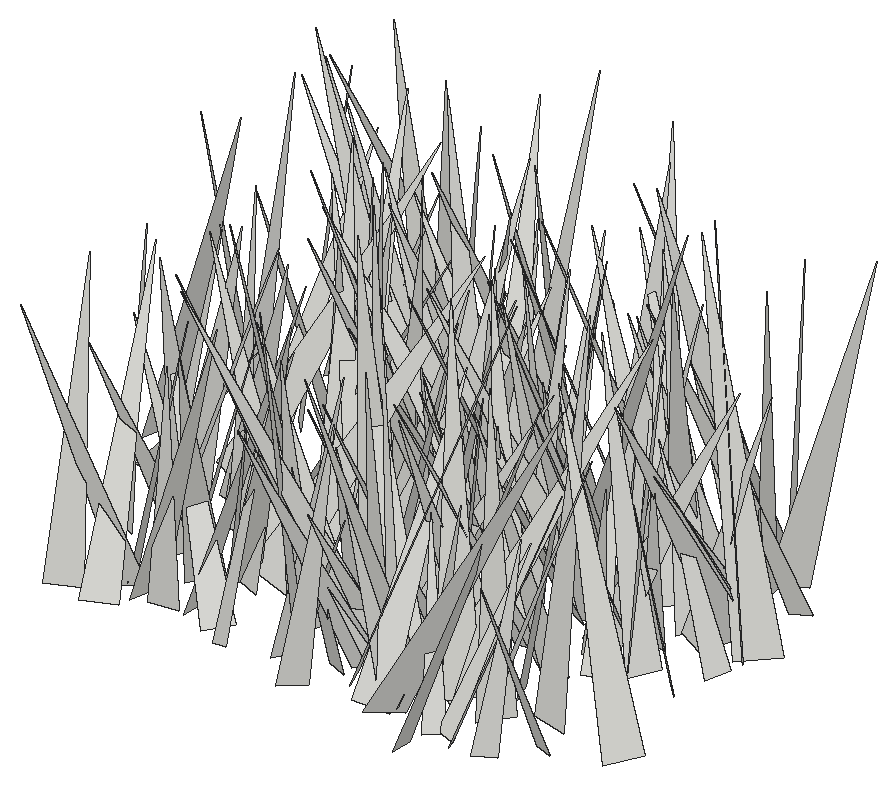
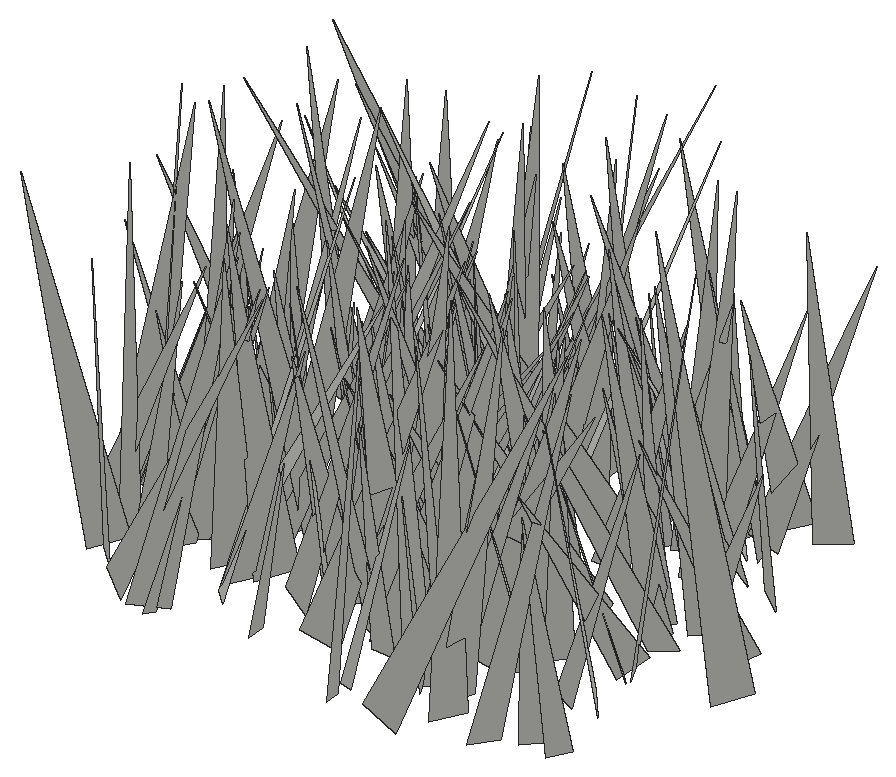
# SketchUp Ruby script. Lengths in inches.
U = 1.inch
M = Sketchup.active_model
def pt(a) = Geom::Point3d.new(a.map { |v| v * U })
def face(e, loops, mat)
  f = e.add_face(loops[0].map { |a| pt(a) })
  loops[1..].each { |l| e.add_face(l.map { |a| pt(a) }).erase! }
  f.material = f.back_material = mat if mat
  f
end
# faces: each face lists its corners as indices into pts; further lists are holes
def faces(e, pts, list, mat = nil) = list.each { |f| face(e, (f[0].is_a?(Array) ? f : [f]).map { |l| l.map { |i| pts[i] } }, mat) }
# xy, xz, yz: faces in a plane at the given z, y or x. An outline is a flat list of corners, or four numbers for a rectangle; further outlines are holes
def ring(l) = l.size == 4 ? [[l[0], l[1]], [l[2], l[1]], [l[2], l[3]], [l[0], l[3]]] : l.each_slice(2).to_a
def flat(e, list, mat, &to3) = list.each { |f| face(e, (f[0].is_a?(Array) ? f : [f]).map { |l| ring(l).map { |u, v| to3.(u, v) } }, mat) }
def xy(e, z, list, mat = nil) = flat(e, list, mat) { |x, y| [x, y, z] }
def xz(e, y, list, mat = nil) = flat(e, list, mat) { |x, z| [x, y, z] }
def yz(e, x, list, mat = nil) = flat(e, list, mat) { |y, z| [x, y, z] }
def lines(e, pts, list) = list.each { |a, b| e.add_line(pt(pts[a]), pt(pts[b])) }
# prism: a flat outline (further loops are holes) pulled along v
def prism(e, loops, v, mat = nil)
  f = face(e, loops, mat); d = Geom::Vector3d.new(v.map { |x| x * U })
  f.pushpull(f.normal.samedirection?(d) ? d.length : -d.length)
end
def box(e, o, s, mat = nil) = prism(e, [[o, [o[0] + s[0], o[1], o[2]], [o[0] + s[0], o[1] + s[1], o[2]], [o[0], o[1] + s[1], o[2]]]], [0, 0, s[2]], mat)
def at(x, y, z, deg = 0) = Geom::Transformation.translation(pt([x, y, z])) * Geom::Transformation.rotation(ORIGIN, Z_AXIS, deg.degrees)
def axes(o, x, y, z) = Geom::Transformation.new([*x, 0, *y, 0, *z, 0, *pt(o).to_a, 1])
def part(name) = M.definitions.add(name)
# library, detail: a bought-in or finely detailed component or shape, given as its bounding box
def library(name, o, s) = part(name).tap { |d| box(d.entities, o, s) }
def detail(e, o, s) = box(e.add_group.entities, o, s)
def put(e, d, t, mat = nil) = e.add_instance(d, t).tap { |i| i.material = mat if mat }
def group(e, t, mat = nil) = e.add_group.tap { |g| g.transformation = t; g.material = mat if mat }.entities
root = M.entities
c1 = part("fur_instance\#9")
p = [[0.8125,0,1.79],[0.67,-0.02,1.48],[0,-0.11,0],[0,0.11,0]]
faces(c1.entities,p,[[0,1,2,3]])
put(root,c1,axes([124.41,342.08,-27.1],[4.29417,-2.87763,1.75823],[-3.19183,-4.38696,0.6155],[-1.08829,1.5119,5.13243]))
put(root,c1,axes([124.15,342.98,-27.1],[-6.04607,-3.24149,2.31572],[-3.3744,6.40425,0.15438],[2.11738,0.95032,6.85845]))
put(root,c1,axes([125.6,344.76,-27.1],[1.43774,-5.64122,0.58152],[-5.34924,-1.54822,-1.79367],[-1.88339,0.09091,5.53834]))
put(root,c1,axes([133.97,343.88,-27.1],[-1.2303,-3.6424,0.32202],[-3.65502,1.23499,0.00478],[0.10759,0.30356,3.84457]))
put(root,c1,axes([132.68,342.28,-27.1],[-2.57998,2.99071,1.64125],[3.02202,2.95835,-0.64026],[1.58287,-0.77341,3.89753]))
put(root,c1,axes([126.14,345.06,-27.1],[-8.04638,-2.10125,0.20494],[-2.02323,7.90531,1.61682],[0.60315,-1.51404,8.15753]))
put(root,c1,axes([127.17,345.21,-27.1],[-6.19203,-3.31038,1.54754],[-2.85802,6.28451,2.00782],[2.2771,-1.114,6.72819]))
put(root,c1,axes([115.82,344.11,-27.1],[-0.4063,-5.76079,1.26429],[-5.69006,0.04941,-1.60344],[-1.5519,1.32705,5.54804]))
put(root,c1,axes([116.51,344.07,-27.1],[6.83641,-1.96558,0.32372],[-1.94381,-6.83529,-0.45298],[-0.43579,-0.34652,7.09893]))
put(root,c1,axes([117.53,343.63,-27.1],[1.49528,-4.80686,1.53266],[-5.04418,-1.45777,0.34917],[-0.10564,1.56838,5.02194]))
put(root,c1,axes([130.01,341.07,-27.1],[6.47636,2.00005,0.90058],[1.74291,-6.39683,1.67254],[-1.33173,1.35459,6.56857]))
put(root,c1,axes([127.65,343.46,-27.1],[-4.79801,0.15244,1.14259],[0.25589,4.91001,0.4195],[1.12396,-0.46714,4.78206]))
put(root,c1,axes([128.04,342.59,-27.1],[7.15691,-3.14413,0.26361],[-3.09126,-6.8566,2.14652],[0.63178,2.06831,7.5166]))
put(root,c1,axes([113.94,342.64,-27.1],[3.27303,-4.65782,3.06275],[-5.40234,-3.52629,0.41046],[-1.37496,2.76738,5.67799]))
put(root,c1,axes([130.34,342.45,-27.1],[-3.13044,2.30171,0.23571],[2.28042,3.13636,-0.34054],[0.39127,0.13578,3.8706]))
put(root,c1,axes([123.11,344.1,-27.1],[3.6641,-0.22277,0.06955],[-0.2117,-3.63329,-0.48425],[-0.09821,-0.47926,3.63879]))
put(root,c1,axes([117.4375,346.02,-27.1],[4.70982,-4.44224,0.12242],[-4.38661,-4.67586,-0.90827],[-0.71149,-0.57769,6.41023]))
put(root,c1,axes([125.21,346.05,-27.1],[3.98276,-1.20965,1.22676],[-0.42908,-3.68899,-2.24451],[-1.66855,-1.93873,3.5054]))
put(root,c1,axes([130.77,342.53,-27.1],[0.96645,3.75371,0.08435],[3.72936,-0.9496,-0.47076],[0.43512,-0.19848,3.84744]))
put(root,c1,axes([128.98,343.77,-27.1],[4.01363,-0.60213,1.19124],[-0.70216,-4.16285,0.26162],[-1.13516,0.446,4.0501]))
put(root,c1,axes([126.4,344.49,-27.1],[5.75232,0.0292,2.58276],[0.25276,-6.28131,-0.49192],[-2.57052,-0.55229,5.73133]))
put(root,c1,axes([122.47,345.18,-27.1],[5.42089,-2.3865,1.81758],[-2.19868,-5.71457,-0.94576],[-2.04078,-0.18248,5.84696]))
put(root,c1,axes([128.19,343.6,-27.1],[5.44846,0.74036,0.07595],[0.73692,-5.44519,0.21553],[-0.10422,0.20337,5.4943]))
put(root,c1,axes([131.22,342.29,-27.1],[4.24517,2.47398,0.29086],[2.34061,-4.15824,1.20716],[-0.85248,0.90284,4.76286]))
put(root,c1,axes([124.87,343.93,-27.1],[-5.12266,-6.1706,2.10185],[-6.50165,4.64284,-2.21548],[-0.47189,3.01719,7.70776]))
put(root,c1,axes([122.875,343.51,-27.1],[5.08359,-0.28901,1.82683],[-0.68576,-5.25683,1.07667],[-1.71772,1.24337,4.97667]))
put(root,c1,axes([131.36,344.55,-27.1],[4.8811,-3.48072,2.77846],[-3.79933,-5.40519,-0.09683],[-2.32386,1.52607,5.99426]))
put(root,c1,axes([131.47,343.63,-27.1],[4.74716,3.3592,0.52437],[3.38285,-4.75689,-0.1518],[-0.33985,-0.42721,5.81349]))
put(root,c1,axes([119.93,343.64,-27.1],[-3.53792,4.34861,0.23075],[4.30519,3.44804,1.02808],[-0.65501,-0.82532,5.51093]))
put(root,c1,axes([127.45,342.58,-27.1],[-1.69129,6.09931,0.73665],[6.01995,1.79783,-1.06428],[1.22654,-0.41345,6.23934]))
put(root,c1,axes([124.03,346.29,-27.1],[4.34393,-1.36952,0.92271],[-1.07858,-4.31928,-1.3331],[-1.25046,-1.03195,4.35524]))
put(root,c1,axes([119.15,345.18,-27.1],[3.83115,1.46002,1.29175],[1.69697,-3.89964,-0.62537],[-0.95945,-1.06731,4.05194]))
put(root,c1,axes([115.32,344.71,-27.1],[5.01565,1.80166,1.23073],[1.89818,-5.12441,-0.23415],[-1.07592,-0.64182,5.32428]))
put(root,c1,axes([122.2,347.21,-27.1],[-5.96811,-4.81477,0.42538],[-4.75156,5.96808,0.88657],[0.88638,-0.42578,7.61672]))
put(root,c1,axes([115.61,342.48,-27.1],[-4.47188,4.60163,0.40246],[4.4512,4.44255,-1.33612],[1.23441,0.65071,6.27595]))
put(root,c1,axes([120.68,342.74,-27.1],[2.07794,4.44656,0.23399],[4.16362,-2.03187,1.63715],[-1.57826,0.49406,4.62704]))
put(root,c1,axes([118.5,346.7,-27.1],[6.88515,-2.28469,0.18682],[-2.24647,-6.84269,-0.88939],[-0.45618,-0.78602,7.19959]))
put(root,c1,axes([115.79,347.21,-27.1],[0.74185,-5.118,0.35857],[-5.01336,-0.80012,-1.04825],[-1.09027,0.19676,5.06413]))
put(root,c1,axes([118.43,344.2,-27.1],[6.55283,1.12937,1.12544],[0.97488,-6.60494,0.95181],[-1.26162,0.76214,6.58096]))
put(root,c1,axes([128.43,347.47,-27.1],[1.50349,-5.86365,0.5049],[-5.82358,-1.55753,-0.74685],[-0.85041,0.2992,6.00709]))
put(root,c1,axes([123.91,345.74,-27.1],[-5.32926,2.77314,1.19327],[2.9808,5.21718,1.1879],[0.47858,-1.6143,5.88899]))
put(root,c1,axes([136.55,345.05,-27.1],[-5.76808,3.66085,1.08427],[3.77252,5.76709,0.59739],[0.58783,-1.08949,6.80556]))
put(root,c1,axes([129.43,344.84,-27.1],[-5.69,4.35692,2.08043],[4.49689,5.95288,-0.16772],[1.75752,-1.1258,7.16454]))
put(root,c1,axes([115.99,347.31,-27.1],[4.78165,-4.93816,1.39024],[-4.88475,-4.96331,-0.82896],[-1.56762,0.40313,6.82367]))
put(root,c1,axes([125.73,343.85,-27.1],[6.75975,3.62956,0.52461],[3.54067,-6.74583,1.04905],[-0.95528,0.68056,7.60048]))
put(root,c1,axes([129.96,348.8,-27.1],[-4.86076,-4.47494,0.06756],[-4.36579,4.76306,1.38194],[0.98465,-0.972,6.46083]))
put(root,c1,axes([127.02,345.13,-27.1],[-4.60264,5.20733,0.96805],[5.29634,4.53648,0.77902],[0.04773,-1.24166,6.90606]))
put(root,c1,axes([127.35,347,-27.1],[-2.08811,-4.65792,0.59921],[-4.45757,1.75934,-1.85749],[-1.47829,1.27435,4.7546]))
put(root,c1,axes([124.63,346.9,-27.1],[-4.81324,5.46383,3.73935],[6.29264,5.21276,0.48307],[2.05886,-3.15867,7.26549]))
put(root,c1,axes([126.47,344.69,-27.1],[1.43872,7.93621,2.15807],[7.82752,-1.99366,2.11323],[-2.52399,-1.65906,7.7838]))
put(root,c1,axes([133.02,345.4,-27.1],[2.04699,7.14679,2.15899],[7.40344,-2.23185,0.36858],[-0.96272,-1.9673,7.42502]))
put(root,c1,axes([118.97,346.43,-27.1],[1.57919,4.13225,1.33364],[4.34025,-1.54395,-0.35548],[-0.12772,-1.37428,4.40942]))
put(root,c1,axes([127.67,347,-27.1],[4.70905,2.28139,1.77217],[2.5251,-4.89691,-0.40574],[-1.40329,-1.15586,5.21682]))
put(root,c1,axes([128.81,344.8,-27.1],[2.72489,7.5123,0.23605],[7.26372,-2.56761,-2.13568],[1.931,-0.94238,7.70056]))
put(root,c1,axes([130.98,348.26,-27.1],[-0.18696,-5.47828,1.21386],[-5.53827,-0.01495,-0.92048],[-0.90141,1.22808,5.40363]))
put(root,c1,axes([116.23,344.57,-27.1],[4.52328,4.39752,0.22155],[4.10164,-4.32376,2.0806],[-1.60118,1.34692,5.95561]))
put(root,c1,axes([123.45,349.17,-27.1],[-3.4189,-2.83051,0.24342],[-2.77437,3.40847,0.66713],[0.61145,-0.36118,4.38812]))
put(root,c1,axes([125.12,348.16,-27.1],[2.82245,-3.27125,1.23973],[-3.47956,-2.78972,0.56063],[-0.36142,1.31172,4.28404]))
put(root,c1,axes([113.125,347.09,-27.1],[2.73063,4.59292,1.67983],[4.59916,-3.06583,0.90635],[-1.66266,-0.93747,5.2659]))
put(root,c1,axes([130.91,346.52,-27.1],[6.22186,3.72093,2.03459],[3.43335,-6.54009,1.46143],[-2.48938,0.27987,7.10078]))
put(root,c1,axes([127.45,348.77,-27.1],[-3.50463,1.38607,1.3282],[1.66931,3.56562,0.68373],[0.94799,-1.15452,3.70623]))
put(root,c1,axes([115.04,346.38,-27.1],[2.36342,5.34352,0.74133],[5.25737,-2.46286,0.99138],[-1.20944,-0.26392,5.75813]))
put(root,c1,axes([114.99,348.9,-27.1],[4.88196,1.64498,0.71636],[1.77456,-4.73338,-1.22423],[-0.26474,-1.39349,5.00407]))
put(root,c1,axes([128.9,349.17,-27.1],[-1.8038,-4.78632,0.84713],[-4.75617,1.55162,-1.36069],[-1.00264,1.25053,4.93062]))
put(root,c1,axes([131.8,351.32,-27.1],[-2.90473,-5.90083,0.221],[-5.68544,2.86131,1.67173],[1.5951,-0.54696,6.36102]))
put(root,c1,axes([125.07,347.5625,-27.1],[2.90433,5.023,0.38727],[4.82562,-2.64532,-1.87916],[1.44702,-1.25991,5.48948]))
put(root,c1,axes([131.39,349.89,-27.1],[0.93641,-4.49496,0.58968],[-4.44892,-0.79539,1.00188],[0.87152,0.76939,4.48082]))
put(root,c1,axes([123.19,348.88,-27.1],[5.83146,1.27805,1.15338],[1.33487,-5.92923,-0.17895],[-1.08712,-0.42484,5.96719]))
put(root,c1,axes([118.87,348.72,-27.1],[-2.86629,5.19134,1.30889],[5.27356,2.48156,1.70596],[-0.92348,-1.94182,5.67938]))
put(root,c1,axes([128.82,351.97,-27.1],[-3.40543,-6.99905,0.02732],[-6.9991,3.40539,-0.01642],[-0.00281,0.03175,7.78353]))
put(root,c1,axes([126.48,350.57,-27.1],[-3.7934,-3.57067,0.95546],[-3.47781,3.9116,0.81037],[1.25196,0.04698,5.14615]))
put(root,c1,axes([119.21,347.23,-27.1],[-0.59602,7.49567,1.64856],[6.68012,1.32078,-3.59019],[3.77872,-1.15261,6.60687]))
put(root,c1,axes([134.82,349.9,-27.1],[-2.53419,-2.69204,0.92744],[-2.77792,2.61003,-0.01451],[0.6248,0.68554,3.69715]))
put(root,c1,axes([115.08,350.74,-27.1],[1.45023,-6.39796,1.08768],[-6.25164,-1.07813,1.99368],[1.74182,1.45734,6.24998]))
put(root,c1,axes([114.0625,349.21,-27.1],[-1.40668,3.30295,0.84871],[3.29754,1.08331,1.24951],[-0.86952,-1.23511,3.36556]))
put(root,c1,axes([129.87,352.19,-27.1],[2.52782,-6.77606,0.30453],[-6.73549,-2.54598,-0.74076],[-0.80053,0.02468,7.19418]))
put(root,c1,axes([113.36,350.26,-27.1],[2.93008,-5.46925,1.49234],[-5.65269,-2.69042,1.23848],[0.43226,1.89052,6.07982]))
put(root,c1,axes([116.31,349.24,-27.1],[1.54209,5.92638,1.72605],[6.04197,-1.81335,0.82809],[-1.2633,-1.43843,6.06748]))
put(root,c1,axes([132.16,348.97,-27.1],[-1.31854,4.49628,0.43937],[4.51767,1.31381,0.11263],[0.01505,-0.45333,4.68427]))
put(root,c1,axes([114.54,351.34,-27.1],[1.31964,-4.20384,0.49444],[-3.9297,-1.02429,1.77946],[1.57296,0.96785,4.03079]))
put(root,c1,axes([111.18,350.72,-27.1],[2.58418,-3.37784,0.00054],[-2.92311,-2.23595,2.1316],[1.69269,1.29557,3.68023]))
put(root,c1,axes([127.53,350.21,-27.1],[-3.57367,4.96866,1.72232],[5.21894,3.60663,0.42422],[0.64547,-1.65218,6.10563]))
put(root,c1,axes([133.32,350.18,-27.1],[-5.60882,2.54428,1.1021],[2.59069,5.69507,0.03704],[0.9881,-0.48955,6.15881]))
put(root,c1,axes([132.29,351.99,-27.1],[0.84886,-4.32385,0.54485],[-4.30912,-0.7498,0.76315],[0.65118,0.6747,4.3398]))
put(root,c1,axes([132.6,350.04,-27.1],[-3.91577,-3.49387,3.17429],[-4.26524,4.38586,-0.43413],[2.02262,2.48468,5.2299]))
put(root,c1,axes([122.07,350.27,-27.1],[-0.00345,4.9845,1.60202],[5.18158,-0.22632,0.71534],[-0.75028,-1.58596,4.93291]))
put(root,c1,axes([134.37,354.1,-27.1],[4.00993,-5.51552,0.33203],[-5.14979,-3.87921,-2.24547],[-2.00271,-1.06842,6.43882]))
put(root,c1,axes([128.66,352.97,-27.1],[-6.87561,-0.89332,0.66489],[-0.69538,6.69239,1.80069],[0.86979,-1.71115,6.69549]))
put(root,c1,axes([131.08,350.51,-27.1],[0.63179,6.0642,2.01169],[5.81387,0.29266,-2.70812],[2.6496,-2.08816,5.46258]))
put(root,c1,axes([126.26,351.95,-27.1],[-2.43401,-4.94438,0.27236],[-4.40728,2.02468,-2.63096],[-2.25763,1.37813,4.84245]))
put(root,c1,axes([125.18,352.21,-27.1],[2.03296,-3.43324,0.36978],[-3.45285,-2.01606,0.26469],[0.04074,0.45292,3.9812]))
put(root,c1,axes([130.52,352.83,-27.1],[-1.29347,-4.18784,0.40951],[-4.17089,1.33267,0.45438],[0.55623,0.25449,4.35943]))
put(root,c1,axes([123.68,351.09,-27.1],[5.7925,1.49056,1.34896],[1.52882,-5.93778,-0.00376],[-1.30544,-0.3399,5.9812]))
put(root,c1,axes([120.92,351.49,-27.1],[-2.66914,2.15187,1.53787],[2.38339,2.90414,0.07299],[1.14676,-1.02728,3.42776]))
put(root,c1,axes([131.25,351.26,-27.1],[-2.34168,-2.41248,1.9117],[-2.76899,2.70012,0.01564],[1.3444,1.35921,3.36204]))
put(root,c1,axes([135.36,351.68,-27.1],[-3.9914,1.89648,0.82188],[2.01712,3.964,0.64912],[0.45094,-0.94526,4.3711]))
put(root,c1,axes([122.61,353.375,-27.1],[-0.7364,-6.55979,0.93298],[-6.36781,0.44127,-1.92351],[-1.83094,1.10364,6.31453]))
put(root,c1,axes([123.43,351.53,-27.1],[-1.82115,-3.36265,1.61921],[-3.73204,1.65736,-0.7556],[0.03439,1.7865,3.74875]))
put(root,c1,axes([120.5,351.44,-27.1],[4.06784,5.47307,2.7985],[5.78633,-4.54195,0.47187],[-2.07475,-1.93641,6.80288]))
put(root,c1,axes([127.06,350.04,-27.1],[-6.05954,0.33778,0.89505],[0.02694,5.79744,-2.00555],[0.95629,1.97708,5.728]))
put(root,c1,axes([109.81,353.3,-27.1],[8.0282,-2.33719,0.44231],[-2.30718,-8.02996,-0.55383],[-0.57877,-0.40914,8.34313]))
put(root,c1,axes([125.32,351.76,-27.1],[-1.86227,-3.58892,1.59018],[-3.91628,1.57852,-1.02377],[-0.26793,1.87217,3.91156]))
put(root,c1,axes([134.66,355.04,-27.1],[-4.06772,-3.26977,0.32403],[-2.78571,3.7053,2.41936],[1.74246,-1.70943,4.62433]))
put(root,c1,axes([119.39,351.01,-27.1],[1.43263,3.39143,0.32506],[3.34277,-1.46736,0.57677],[-0.65831,-0.07043,3.63615]))
put(root,c1,axes([123.82,353.3,-27.1],[4.04014,-3.74392,1.13553],[-3.80741,-4.13804,-0.09691],[-0.90002,0.69913,5.50729]))
put(root,c1,axes([113.61,353.96,-27.1],[-6.01698,-4.0059,2.23214],[-3.85326,6.41302,1.12219],[2.48637,0.24439,7.14087]))
put(root,c1,axes([127.23,351.57,-27.1],[1.06492,5.99669,1.55027],[6.17359,-1.15473,0.22589],[-0.50038,-1.48458,6.08632]))
put(root,c1,axes([122.11,353.65,-27.1],[-5.99234,-4.15881,0.58341],[-4.19764,5.96205,-0.6148],[0.12593,0.83815,7.26814]))
put(root,c1,axes([119.22,350.88,-27.1],[-5.83364,4.02968,1.05878],[3.90844,5.92385,-1.01134],[1.44341,0.24573,7.01761]))
put(root,c1,axes([120.09,351.58,-27.1],[-5.57386,3.34507,0.61319],[3.34749,5.6042,-0.14346],[0.5998,-0.19191,6.49898]))
put(root,c1,axes([118.17,353.05,-27.1],[5.45486,-2.53583,1.72286],[-2.73109,-5.61705,0.37948],[-1.39279,1.08278,6.00349]))
put(root,c1,axes([126.59,353.8,-27.1],[0.40641,-5.35004,1.66525],[-5.54368,-0.62666,-0.66032],[-0.81458,1.59547,5.32467]))
put(root,c1,axes([115.12,350.8,-27.1],[-7.30658,0.78889,2.52937],[0.00726,7.42557,-2.29501],[2.64953,2.15518,6.98151]))
put(root,c1,axes([126.48,354.3,-27.1],[4.42301,-0.66017,1.25029],[-0.31732,-4.46498,-1.23502],[-1.37781,-1.09094,4.29808]))
put(root,c1,axes([123.5,354.47,-27.1],[-6.69596,1.51903,0.23584],[1.52209,6.40398,1.96756],[-0.2152,-1.96993,6.57815]))
put(root,c1,axes([123.33,350.55,-27.1],[1.15921,7.66569,0.40932],[7.66684,-1.17697,0.3294],[-0.3873,-0.35503,7.74584]))
put(root,c1,axes([125.68,352.76,-27.1],[2.94995,3.39967,1.09614],[3.50655,-3.02709,-0.04841],[-0.68072,-0.86052,4.50085]))
put(root,c1,axes([116.93,351.48,-27.1],[5.85572,0.96623,0.0245],[0.91904,-5.61274,1.69591],[-0.29926,1.66948,5.68743]))
put(root,c1,axes([120.04,353.47,-27.1],[-0.77614,4.62516,2.62163],[4.88719,1.66369,-1.48826],[2.09294,-2.16967,4.44742]))
put(root,c1,axes([130.79,355.67,-27.1],[0.39282,-7.92697,1.06347],[-7.86049,-0.18606,1.51663],[1.47665,1.11832,7.79044]))
put(root,c1,axes([127.57,353.51,-27.1],[8.28106,0.30024,0.90595],[0.31898,-8.32832,-0.15571],[-0.89952,-0.18935,8.28504]))
put(root,c1,axes([133.2,352.92,-27.1],[2.00403,4.77087,1.2081],[4.88814,-1.77806,-1.08691],[0.57161,-1.52123,5.05925]))
put(root,c1,axes([116.21,354.83,-27.1],[5.02867,-2.50397,0.95955],[-2.41233,-5.11484,-0.70513],[-1.17101,-0.21602,5.57317]))
put(root,c1,axes([128.75,354.52,-27.1],[-2.94744,-5.34651,0.76174],[-5.29498,2.69026,-1.60576],[-1.06233,1.42484,5.89017]))
put(root,c1,axes([135.75,353.45,-27.1],[-4.55755,6.1935,2.40469],[6.62517,4.45559,1.08074],[0.49905,-2.58872,7.61332]))
put(root,c1,axes([135.03,353.36,-27.1],[-5.85102,-5.01294,3.05498],[-5.59861,6.06235,-0.77491],[1.76582,2.61061,7.66574]))
put(root,c1,axes([113.83,352.07,-27.1],[1.59933,7.72158,1.03232],[7.26868,-1.09996,-3.03359],[2.80263,-1.55359,7.2786]))
put(root,c1,axes([120.22,353.97,-27.1],[4.77754,4.17311,2.72058],[4.61145,-5.13068,-0.22808],[-1.8844,-1.97551,6.33938]))
put(root,c1,axes([119.35,351.13,-27.1],[-1.39232,7.88876,0.40308],[7.89477,1.37627,0.33483],[-0.26016,-0.45487,8.00369]))
put(root,c1,axes([118.83,355.16,-27.1],[0.4901,-6.09421,1.40714],[-6.12992,-0.18765,1.32232],[1.24239,1.47818,5.96918]))
put(root,c1,axes([120.79,352.09,-27.1],[-3.36626,3.2291,1.55087],[2.48228,3.63709,-2.18492],[2.58275,0.71309,4.12128]))
put(root,c1,axes([131.17,351.56,-27.1],[3.09687,5.17866,0.3937],[4.90573,-3.06729,1.75775],[-1.70508,0.58082,5.7723]))
put(root,c1,axes([132.82,353.65,-27.1],[-6.31107,2.62453,1.38258],[2.63294,6.45317,-0.23139],[1.36651,-0.31261,6.83112]))
put(root,c1,axes([122.08,354.78,-27.1],[2.26565,-5.57265,3.25786],[-5.77256,-3.29433,-1.62055],[-2.88887,2.21229,5.79322]))
put(root,c1,axes([113.57,354.49,-27.1],[3.56732,3.05528,0.6125],[3.0981,-3.37772,-1.19517],[0.33415,-1.30074,4.54225]))
put(root,c1,axes([123.37,353.85,-27.1],[-7.4138,3.10521,1.79195],[3.13289,7.61249,-0.22981],[1.74312,-0.47482,8.03455]))
put(root,c1,axes([122.11,352.8,-27.1],[-0.74484,5.04348,0.31723],[4.84937,0.80355,-1.38926],[1.42161,-0.09859,4.90524]))
put(root,c1,axes([121.17,356.03,-27.1],[2.55159,-4.81811,0.15811],[-4.66384,-2.42197,1.46026],[1.21971,0.81832,5.25284]))
put(root,c1,axes([116.51,356.14,-27.1],[4.04472,-2.80495,1.23292],[-2.68281,-4.22845,-0.81868],[-1.47998,-0.00072,4.85358]))
put(root,c1,axes([130.94,354.36,-27.1],[-3.74669,3.50171,1.17991],[3.59906,3.83892,0.03541],[0.8372,-0.8322,5.12819]))
put(root,c1,axes([129.78,355.3,-27.1],[-5.18196,-4.15409,0.26027],[-4.02731,4.89921,-1.98883],[-1.05116,1.70828,6.3367]))
put(root,c1,axes([125.33,355.01,-27.1],[-5.00491,-0.78513,1.46412],[-0.94309,5.16869,-0.45214],[1.36772,0.69095,5.0459]))
put(root,c1,axes([117.93,353.81,-27.1],[-5.27031,-0.93158,1.82448],[-1.52104,5.15288,-1.7627],[1.37223,2.13373,5.05341]))
put(root,c1,axes([121.33,357.66,-27.1],[3.93068,-5.30389,1.53813],[-4.85639,-4.21869,-2.1367],[-2.62918,-0.13704,6.24628]))
put(root,c1,axes([132.51,357.03,-27.1],[3.93846,-2.19121,0.70559],[-1.95473,-3.92185,-1.26841],[-1.21585,-0.79274,4.32481]))
put(root,c1,axes([134.93,356.78,-27.1],[-0.6126,-5.21006,0.97224],[-5.10965,0.32064,-1.50131],[-1.40764,1.1035,5.02654]))
put(root,c1,axes([127.97,358.625,-27.1],[-5.57338,-5.53642,0.81265],[-5.27737,5.58191,1.83481],[1.86058,-0.75178,7.63858]))
put(root,c1,axes([124.06,356.1,-27.1],[-6.12139,2.10353,0.29479],[2.12072,6.0019,1.20952],[-0.1196,-1.23917,6.35872]))
put(root,c1,axes([131.29,356.63,-27.1],[-5.2528,1.04607,1.18822],[1.28573,5.22141,1.0871],[0.92359,-1.31932,5.24446]))
put(root,c1,axes([131.82,356.56,-27.1],[-5.37487,-0.5228,0.79074],[-0.44432,5.41107,0.55741],[0.83736,-0.48456,5.37139]))
put(root,c1,axes([114.31,356.93,-27.1],[-1.82389,-4.57282,0.8897],[-4.65371,1.74485,-0.5721],[-0.21262,1.03617,4.88978]))
put(root,c1,axes([133.42,356.84,-27.1],[6.36794,0.62079,2.33056],[0.97414,-6.68136,-0.88201],[-2.20634,-1.15823,6.33704]))
put(root,c1,axes([123.21,355.0625,-27.1],[-4.28711,2.60894,1.39768],[2.40918,4.50508,-1.01958],[1.71929,0.19268,4.91389]))
put(root,c1,axes([119.54,355.68,-27.1],[3.95352,-1.35205,0.74696],[-1.51739,-3.78343,1.18299],[-0.28899,1.3689,4.00736]))
put(root,c1,axes([118.78,359.24,-27.1],[8.12463,-0.31909,0.21051],[-0.21684,-7.53553,-3.0536],[-0.31483,-3.04462,7.53571]))
put(root,c1,axes([123.47,358.88,-27.1],[0.28426,-7.43419,0.75555],[-7.30944,-0.43371,-1.51752],[-1.55247,0.68085,7.28321]))
put(root,c1,axes([125.8,357.24,-27.1],[-3.53449,-6.31522,1.62159],[-6.50822,3.306,-1.31053],[-0.39309,2.04757,7.11738]))
put(root,c1,axes([125.5,355.1875,-27.1],[-4.48164,3.41054,1.04148],[3.17852,4.57879,-1.31654],[1.61662,0.45221,5.47573]))
put(root,c1,axes([131.28,356.12,-27.1],[-5.13567,3.95215,0.39173],[3.97037,5.09374,0.66187],[-0.09557,-0.76314,6.44644]))
put(root,c1,axes([123.96,357.56,-27.1],[4.93042,2.67254,1.54888],[2.99605,-4.84755,-1.1728],[-0.75178,-1.79146,5.48417]))
put(root,c1,axes([118.12,356.65,-27.1],[-2.53782,7.33959,2.16761],[7.45924,1.86167,2.42953],[-1.71111,-2.77006,7.37615]))
put(root,c1,axes([113.84,353.73,-27.1],[-4.95607,3.58078,0.35964],[3.00453,4.45388,-2.94106],[1.98095,2.2034,5.36049]))
put(root,c1,axes([120.14,356.14,-27.1],[-2.8355,7.09509,0.7949],[6.33308,2.10473,3.80453],[-3.2961,-2.05963,6.62616]))
put(root,c1,axes([127.45,356.22,-27.1],[5.828,-3.21448,3.45143],[-4.0564,-6.21538,1.06086],[-2.40642,2.69201,6.57061]))
put(root,c1,axes([122.92,355.14,-27.1],[-3.64093,6.72533,0.73654],[6.73348,3.68347,-0.34805],[0.65778,-0.48058,7.63972]))
put(root,c1,axes([118.45,357.79,-27.1],[-6.63907,0.80935,0.83748],[0.8673,6.67065,0.42894],[0.7773,-0.53025,6.67446]))
put(root,c1,axes([119.55,357.06,-27.1],[-5.60874,-1.91132,2.91151],[-2.48414,6.06379,-0.80475],[2.44113,1.77916,5.87056]))
put(root,c1,axes([128.22,357.42,-27.1],[-5.4054,2.23783,0.44972],[2.26041,5.40869,0.2551],[0.31726,-0.40826,5.84475]))
put(root,c1,axes([113.28,356.39,-27.1],[4.45887,4.52554,1.75159],[4.30275,-4.78695,1.41478],[-2.24387,-0.18639,6.19358]))
put(root,c1,axes([113.875,358.39,-27.1],[4.52674,3.32324,0.78926],[3.39525,-4.2348,-1.64226],[0.37301,-1.78348,5.37013]))
put(root,c1,axes([133.36,358.06,-27.1],[5.70203,-3.94241,1.833],[-4.2894,-5.59456,1.31056],[-0.70959,2.13867,6.80721]))
put(root,c1,axes([129.09,356.48,-27.1],[5.10712,-2.96498,5.20518],[-4.57955,-6.3419,0.88079],[-3.86171,3.59957,5.83935]))
put(root,c1,axes([129.23,361,-27.1],[-5.21619,-2.22313,1.39253],[-1.54183,5.10575,2.37575],[2.12232,-1.75473,5.14847]))
put(root,c1,axes([121.18,358.24,-27.1],[0.37459,4.6587,1.44665],[4.87681,-0.39143,-0.00226],[-0.11359,-1.44218,4.67373]))
put(root,c1,axes([120.75,360.82,-27.1],[-2.24525,-3.81491,0.32062],[-3.67914,2.25292,1.04201],[1.05843,-0.26136,4.3022]))
put(root,c1,axes([116.68,360.29,-27.1],[7.00851,-2.19777,2.01204],[-2.01969,-7.2848,-0.92211],[-2.19075,-0.31499,7.28692]))
put(root,c1,axes([129.54,360.66,-27.1],[4.80769,-4.80499,2.60276],[-4.52111,-5.44469,-1.70033],[-3.0695,0.49361,6.58109]))
put(root,c1,axes([132.78,358.875,-27.1],[3.82157,4.19761,2.25189],[4.45533,-4.17126,0.21447],[-1.68552,-1.50865,5.67259]))
put(root,c1,axes([117.2,359.24,-27.1],[-7.37907,1.498,2.27835],[1.63074,7.6926,0.22378],[2.18531,-0.6822,7.52626]))
put(root,c1,axes([121.88,357.61,-27.1],[2.95959,7.19025,1.54721],[7.29869,-3.07695,0.338],[-0.90704,-1.29822,7.76818]))
put(root,c1,axes([113.28,359.99,-27.1],[2.68413,-2.59886,0.79499],[-2.66781,-2.73276,0.07385],[-0.51851,0.60713,3.7354]))
put(root,c1,axes([112.07,359.97,-27.1],[3.6262,-2.26105,0.60128],[-2.31235,-3.63241,0.28605],[-0.35624,0.56255,4.26378]))
put(root,c1,axes([131.46,360.16,-27.1],[-4.03956,-5.75099,0.92293],[-5.66396,3.6166,-2.25467],[-1.3584,2.0224,6.65646]))
put(root,c1,axes([114.64,360.89,-27.1],[-6.49711,1.14641,2.18071],[1.63194,6.61021,1.38712],[1.84567,-1.80917,6.45001]))
put(root,c1,axes([118.75,359.13,-27.1],[-3.28983,-1.54802,1.9149],[-2.00034,3.5437,-0.57187],[1.43591,1.38997,3.59058]))
put(root,c1,axes([118.43,361.89,-27.1],[-1.35129,-7.71927,0.81651],[-7.46816,1.06686,-2.27338],[-2.11671,1.16382,7.49966]))
put(root,c1,axes([125.51,359.79,-27.1],[-3.60239,-0.15597,0.87969],[-0.19043,3.7046,-0.12301],[0.87288,0.16452,3.60367]))
put(root,c1,axes([120.625,361.71,-27.1],[5.99792,1.55177,2.60045],[2.40829,-5.94226,-2.00876],[-1.83589,-2.72525,5.86071]))
